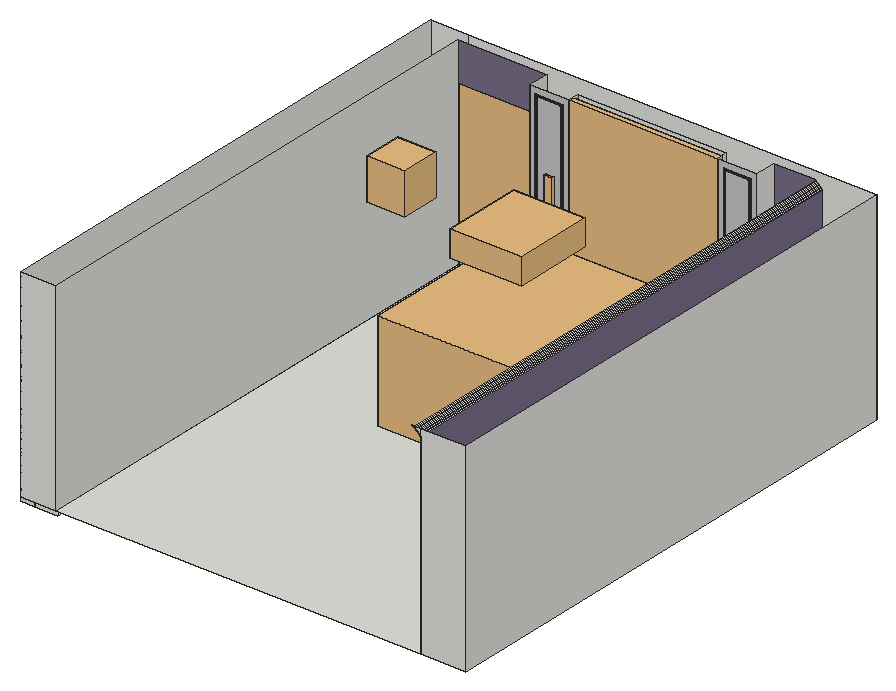
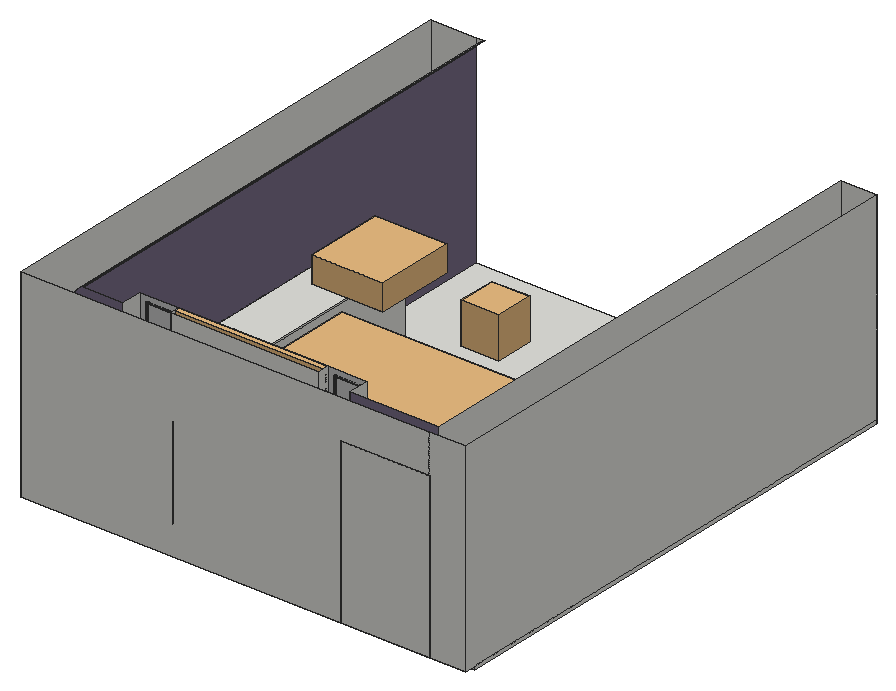
# SketchUp Ruby script. Lengths in inches.
U = 1.inch
M = Sketchup.active_model
def pt(a) = Geom::Point3d.new(a.map { |v| v * U })
def face(e, loops, mat)
  f = e.add_face(loops[0].map { |a| pt(a) })
  loops[1..].each { |l| e.add_face(l.map { |a| pt(a) }).erase! }
  f.material = f.back_material = mat if mat
  f
end
# faces: each face lists its corners as indices into pts; further lists are holes
def faces(e, pts, list, mat = nil) = list.each { |f| face(e, (f[0].is_a?(Array) ? f : [f]).map { |l| l.map { |i| pts[i] } }, mat) }
# xy, xz, yz: faces in a plane at the given z, y or x. An outline is a flat list of corners, or four numbers for a rectangle; further outlines are holes
def ring(l) = l.size == 4 ? [[l[0], l[1]], [l[2], l[1]], [l[2], l[3]], [l[0], l[3]]] : l.each_slice(2).to_a
def flat(e, list, mat, &to3) = list.each { |f| face(e, (f[0].is_a?(Array) ? f : [f]).map { |l| ring(l).map { |u, v| to3.(u, v) } }, mat) }
def xy(e, z, list, mat = nil) = flat(e, list, mat) { |x, y| [x, y, z] }
def xz(e, y, list, mat = nil) = flat(e, list, mat) { |x, z| [x, y, z] }
def yz(e, x, list, mat = nil) = flat(e, list, mat) { |y, z| [x, y, z] }
def lines(e, pts, list) = list.each { |a, b| e.add_line(pt(pts[a]), pt(pts[b])) }
# prism: a flat outline (further loops are holes) pulled along v
def prism(e, loops, v, mat = nil)
  f = face(e, loops, mat); d = Geom::Vector3d.new(v.map { |x| x * U })
  f.pushpull(f.normal.samedirection?(d) ? d.length : -d.length)
end
def box(e, o, s, mat = nil) = prism(e, [[o, [o[0] + s[0], o[1], o[2]], [o[0] + s[0], o[1] + s[1], o[2]], [o[0], o[1] + s[1], o[2]]]], [0, 0, s[2]], mat)
def at(x, y, z, deg = 0) = Geom::Transformation.translation(pt([x, y, z])) * Geom::Transformation.rotation(ORIGIN, Z_AXIS, deg.degrees)
def axes(o, x, y, z) = Geom::Transformation.new([*x, 0, *y, 0, *z, 0, *pt(o).to_a, 1])
def part(name) = M.definitions.add(name)
# library, detail: a bought-in or finely detailed component or shape, given as its bounding box
def library(name, o, s) = part(name).tap { |d| box(d.entities, o, s) }
def detail(e, o, s) = box(e.add_group.entities, o, s)
def put(e, d, t, mat = nil) = e.add_instance(d, t).tap { |i| i.material = mat if mat }
def group(e, t, mat = nil) = e.add_group.tap { |g| g.transformation = t; g.material = mat if mat }.entities
root = M.entities
M.materials.add("[0116_Lavender]").color = [230, 230, 250]
M.materials.add("[Color J01]2").color = [122, 110, 137]
M.materials.add("[Color M01]").color = [226, 226, 226]
M.materials.add("[Color M02]").color = [198, 198, 198]
M.materials.add("[Color M07]").color = [58, 58, 58]
M.materials.add("[Color M08]").color = [30, 30, 30]
c1 = library("Group\#22",[0,-0.85,0],[159.52,154.66,89.09])
c2 = library("Group\#1",[0,0,0],[152.125,5.875,206.4375])
c3 = library("Untitled (23)",[0,0,0],[36,4.39,84])
c4 = part("Group\#46")
prism(c4.entities,[[[0.55,0,1.11],[0.51,0,1.03],[0.44,0,0.97],[0.36,0,0.9375],[0.28,0,0.92],[0.19,0,0.9375],[0.11,0,0.97],[0.05,0,1.03],[0,0,1.11],[0,0,0],[0.55,0,0]]],[0,0.79,0])
c5 = part("Cabinet pull")
put(c5.entities,c4,axes([0,1.42,1.36],[0,0,-1],[1,0,0],[0,-1,0]),"[Color M08]")
g1 = group(c5.entities,at(0,1.42,1.36),"[Color M08]")
prism(g1,[[[0,-1.28,-0.57],[0,-1.32,-0.53],[0,-1.35,-0.49],[0,-1.38,-0.4375],[0,-1.4,-0.39],[0,-1.41,-0.33],[0,-1.42,-0.28],[0,-1.41,-0.22],[0,-1.4,-0.17],[0,-1.38,-0.11],[0,-1.35,-0.0625],[0,-1.32,-0.02],[0,-1.28,0.02],[0,-1.19,0.02],[0,-1.11,0],[0,-1.03,-0.05],[0,-0.97,-0.11],[0,-0.9375,-0.19],[0,-0.92,-0.28],[0,-0.9375,-0.36],[0,-0.97,-0.44],[0,-1.03,-0.51],[0,-1.11,-0.55],[0,-1.19,-0.57]]],[13.07,0,0])
put(c5.entities,c4,axes([12.28,1.42,1.36],[0,0,-1],[1,0,0],[0,-1,0]),"[Color M08]")
c6 = library("Group\#4",[0,0,0],[7.875,1.97,51.61])
c7 = library("Bathroom accessory set",[0,0,0],[18.8125,6.58,10.0625])
c8 = library("lamp",[0,0,0],[9.82,9.84,19.44])
c9 = library("Tabletop vanity mirror",[-0.04,0,0],[13.32,7.875,17.05])
c10 = library("Perfume bottle",[0,0,0],[5.52,3.68,7.92])
c11 = library("Pendant lamp Queen P0244",[-19.36,-19.5625,0],[38.72,39.125,72.84])
c12 = library("031_FANZART_Zen",[-27.59,-27.12,5.07],[46.53,51.77,17.09])
xy(root,-3.875,[[0,0,38.125,513.375]])
xy(root,0,[[0,0,14.41,513.375],[14.41,0,36.34,513.375],[36.34,0,409.59,0,409.59,513.375,359.78,513.375,359.78,491.75,319.78,491.75,319.78,502.75,167.66,502.75,167.66,491.75,127.66,491.75,127.66,524.91,36.34,524.91],[409.59,0,455.6875,0,455.6875,524.91,127.66,524.91,127.66,491.75,167.66,491.75,167.66,502.75,319.78,502.75,319.78,491.75,359.78,491.75,359.78,513.375,409.59,513.375],[0,513.375,36.34,524.91]])
xy(root,4,[[355.03,159.1875,409.59,466.85]])
xy(root,87.5625,[[355.03,159.1875,409.59,466.85]])
xy(root,89.5625,[[355.03,159.1875,409.59,466.85]])
xy(root,166.72,[[36.34,513.375,127.66,524.91]])
xy(root,200.41,[[133.68,491.52,161.63,491.52,161.625,491.75,133.6875,491.75]])
xz(root,0,[[0,-3.875,14.41,0],[14.41,-3.875,38.125,0],[0,0,36.34,206.4375],[409.59,0,455.6875,206.4375],[409.59,198.52,409.59,206.4375,400.78,206.4375,401.6875,206.01,402.57,205.53,403.43,205.01,404.25,204.4375,405.05,203.83,405.8125,203.18,406.54,202.49,407.23,201.76,407.89,201,408.5,200.2,409.07,199.38]])
xz(root,159.1875,[[355.03,4,409.59,87.5625],[355.03,87.5625,409.59,89.5625]])
xz(root,466.85,[[355.03,4,409.59,87.5625],[355.03,87.5625,409.59,89.5625]])
xz(root,491.75,[[[127.66,0,167.66,206.4375],[133.6875,6.03,161.625,200.41]],[[319.78,0,359.78,206.4375],[326.02,6.24,353.54,200.2]],[135.25,7.59,160.0625,198.84],[327.71,7.93,351.86,198.51]],"[Color M02]")
xz(root,502.75,[[167.66,0,319.78,206.4375]])
xz(root,513.375,[[0,-3.875,14.41,0]])
xz(root,513.375,[[359.78,0,409.59,0,409.59,198.52,409.07,199.38,408.5,200.2,407.89,201,407.23,201.76,406.54,202.49,405.8125,203.18,405.05,203.83,404.25,204.4375,403.43,205.01,402.57,205.53,401.6875,206.01,400.78,206.4375,359.78,206.4375],[36.34,166.72,127.66,206.4375]],"[Color J01]2")
xz(root,524.91,[[0,0,0,206.4375,38.125,206.4375,38.125,166.72,36.34,166.72,36.34,0],[36.34,0,127.66,166.72],[127.66,0,127.66,166.72,38.125,166.72,38.125,206.4375,455.6875,206.4375,455.6875,0]])
yz(root,0,[[0,-3.875,513.375,0],[0,0,524.91,206.4375]])
yz(root,14.41,[[0,-3.875,513.375,0]])
yz(root,36.34,[[0,0,524.91,0,524.91,166.72,513.375,166.72,513.375,206.4375,0,206.4375]])
yz(root,127.66,[[491.75,0,491.75,206.4375,513.375,206.4375,513.375,166.72,524.91,166.72,524.91,0]])
yz(root,167.66,[[491.75,0,502.75,206.4375]])
yz(root,319.78,[[491.75,0,502.75,206.4375]])
yz(root,355.03,[[159.1875,4,350.16,87.5625],[408.5,4,466.85,87.5625],[159.1875,87.5625,350.16,89.5625],[350.16,87.5625,408.5,89.5625],[408.5,87.5625,466.85,89.5625]])
yz(root,355.03,[[350.16,4,408.5,24.02],[350.16,24.89,408.5,44.91],[350.16,45.78,408.5,65.8],[350.16,66.67,408.5,86.39]],"[Color J01]2")
yz(root,355.03,[[350.16,24.02,408.5,24.89],[350.16,44.91,408.5,45.78],[350.16,65.8,408.5,66.67],[350.16,86.39,408.5,87.5625]],"[Color M07]")
yz(root,359.78,[[491.75,0,513.375,206.4375]])
yz(root,409.59,[[159.1875,87.5625,466.85,89.5625]])
yz(root,409.59,[[[0,0,513.375,198.52],[159.1875,4,466.85,89.5625]]],"[Color J01]2")
yz(root,455.6875,[[0,0,524.91,206.4375]])
p = [[133.68,491.52,6.02],[133.74,491.29,6.08],[133.74,491.29,200.35],[133.68,491.52,200.41],[161.63,491.52,6.02],[161.57,491.29,6.08],
  [161.63,491.52,200.41],[161.57,491.29,200.35],[133.6875,491.75,6.03],[133.6875,491.75,200.41],[161.625,491.75,6.03],[161.625,491.75,200.41],
  [133.86,491.1,6.2],[133.86,491.1,200.23],[161.45,491.1,6.2],[161.45,491.1,200.23],[134.03,490.94,6.375],[134.03,490.94,200.0625],
  [161.28,490.94,6.375],[161.28,490.94,200.0625],[326.02,491.75,6.24],[326.05,491.53,6.27],[326.05,491.53,200.17],[326.02,491.75,200.2],
  [353.54,491.75,6.24],[353.51,491.53,6.27],[327.71,491.53,6.27],[327.71,491.75,6.24],[353.54,491.75,200.2],[353.51,491.53,200.17],
  [326.13,491.33,6.35],[326.13,491.33,200.09],[327.71,491.33,6.35],[353.43,491.33,6.35],[353.43,491.33,200.09],[134.24,490.85,6.58],
  [134.24,490.85,199.85],[161.07,490.85,6.58],[161.07,490.85,199.85],[326.27,491.15,6.49],[326.27,491.15,199.95],[327.71,491.15,6.49],
  [353.3,491.15,6.49],[353.3,491.15,199.95],[326.44,491.02,6.66],[326.44,491.02,199.78],[353.12,491.02,6.66],[327.71,491.02,6.66],
  [353.12,491.02,199.78],[134.47,490.8125,6.8125],[134.47,490.8125,199.625],[160.84,490.8125,6.8125],[160.84,490.8125,199.625],[326.65,490.93,6.86],
  [326.65,490.93,199.57],[352.92,490.93,6.86],[327.71,490.93,6.86],[352.92,490.93,199.57],[134.7,490.85,7.04],[134.7,490.85,199.4],
  [160.61,490.85,7.04],[160.61,490.85,199.4],[326.86,490.91,7.08],[326.86,490.91,199.36],[352.7,490.91,7.08],[327.71,490.91,7.08],
  [352.7,490.91,199.36],[134.91,490.94,7.25],[134.91,490.94,199.1875],[160.4,490.94,7.25],[160.4,490.94,199.1875],[327.08,490.93,7.3],
  [327.08,490.93,199.14],[352.48,490.93,7.3],[327.71,490.93,7.3],[352.48,490.93,199.14],[135.08,491.1,7.42],[135.08,491.1,199.01],
  [160.23,491.1,7.42],[160.23,491.1,199.01],[327.29,491.02,7.5],[327.29,491.02,198.93],[352.28,491.02,7.5],[327.71,491.02,7.5],
  [352.28,491.02,198.93],[135.2,491.29,7.54],[135.2,491.29,198.89],[160.11,491.29,7.54],[160.11,491.29,198.89],[327.46,491.15,7.68],
  [327.46,491.15,198.76],[352.1,491.15,7.68],[327.71,491.15,7.68],[352.1,491.15,198.76],[135.26,491.52,7.6],[135.26,491.52,198.83],
  [160.05,491.52,7.6],[160.05,491.52,198.83],[135.25,491.75,7.59],[135.25,491.75,198.84],[160.0625,491.75,7.59],[160.0625,491.75,198.84],
  [327.59,491.33,7.8125],[327.59,491.33,198.625],[351.97,491.33,7.8125],[327.71,491.33,7.8125],[351.97,491.33,198.625],[327.68,491.53,7.9],
  [327.68,491.53,198.54],[327.71,491.53,7.9],[351.88,491.53,7.9],[351.88,491.53,198.54],[327.71,491.75,7.93],[327.71,491.75,198.51],
  [351.86,491.75,7.93],[351.86,491.75,198.51],[409.07,513.375,199.38],[409.59,513.375,198.52],[409.59,0,198.52],[409.07,0,199.38],
  [408.5,513.375,200.2],[408.5,0,200.2],[407.89,513.375,201],[407.89,0,201],[407.23,513.375,201.76],[407.23,0,201.76],
  [406.54,513.375,202.49],[406.54,0,202.49],[405.8125,513.375,203.18],[405.8125,0,203.18],[405.05,513.375,203.83],[405.05,0,203.83],
  [404.25,513.375,204.4375],[404.25,0,204.4375],[403.43,513.375,205.01],[403.43,0,205.01],[402.57,513.375,205.53],[402.57,0,205.53]]
faces(root,p,[[0,1,2,3],[4,5,1,0],[8,0,3,9],[10,4,0,8],[1,12,13,2],[5,14,12,1],[12,16,17,13],[14,18,16,12],
  [24,25,26,21,20,27],[32,30,21,26,25,33],[16,35,36,17],[18,37,35,16],[41,39,30,32,33,42],[42,46,47,44,39,41],[35,49,50,36],[37,51,49,35],
  [46,55,56,53,44,47],[49,58,59,50],[51,60,58,49],[55,64,65,62,53,56],[58,67,68,59],[60,69,67,58],[64,73,74,71,62,65],[67,76,77,68],
  [69,78,76,67],[73,82,83,80,71,74],[76,85,86,77],[78,87,85,76],[82,91,92,89,80,83],[85,94,95,86],[87,96,94,85],[94,98,99,95],
  [96,100,98,94],[91,104,105,102,89,92],[109,107,102,105,104,110],[112,107,109,110,114],[116,117,118,119],[103,108,111,106],[108,113,115,111],[90,103,106,93],
  [81,90,93,84],[86,95,97,88],[95,99,101,97],[72,81,84,75],[77,86,88,79],[68,77,79,70],[63,72,75,66],[59,68,70,61],
  [120,116,119,121],[50,59,61,52],[54,63,66,57],[36,50,52,38],[45,54,57,48],[40,45,48,43],[17,36,38,19],[31,40,43,34],
  [13,17,19,15],[22,31,34,29],[122,120,121,123],[2,13,15,7],[23,22,29,28],[3,2,7,6],[124,122,123,125],[126,124,125,127],
  [128,126,127,129],[130,128,129,131],[132,130,131,133],[134,132,133,135],[136,134,135,137]])
faces(root,p,[[6,7,5,4],[11,6,4,10],[7,15,14,5],[15,19,18,14],[19,38,37,18],[38,52,51,37],[52,61,60,51],[61,70,69,60],
  [70,79,78,69],[79,88,87,78],[88,97,96,87],[97,101,100,96]],"[Color M01]")
faces(root,p,[[20,21,22,23],[21,30,31,22],[30,39,40,31],[39,44,45,40],[44,53,54,45],[53,62,63,54],[62,71,72,63],[71,80,81,72],
  [80,89,90,81],[89,102,103,90],[102,107,108,103],[107,112,113,108]],"[Color M02]")
faces(root,p,[[28,29,25,24],[29,34,33,25],[34,43,42,33],[43,48,46,42],[48,57,55,46],[57,66,64,55],[66,75,73,64],[75,84,82,73],
  [84,93,91,82],[93,106,104,91],[106,111,110,104],[111,115,114,110]],"[0116_Lavender]")
put(root,c1,axes([150.38,269.97,0],[1.1342,0,0],[0,1.1342,0],[0,0,1.1342]))
put(root,c2,at(167.66,491.75,0),"[Color M02]")
put(root,c3,axes([37.06,514.75,0],[2.51667,0,0],[0,1,0],[0,0,1.9847]))
put(root,c5,at(353.61,385.24,22.65,-90))
put(root,c5,at(353.61,385.24,43.47,-90))
put(root,c5,at(353.61,385.24,64.47,-90))
put(root,c6,at(334.75,488.35,76.14))
put(root,c6,at(143.99,489.78,79.24))
put(root,c5,at(353.61,385.24,85.22,-90))
put(root,c7,axes([378.68,376.48,89.55],[0,-1.02,0],[1.02,0,0],[0,0,1.02]))
put(root,c8,axes([357.3,424.95,89.5625],[2.4674,0,0],[0,2.4674,0],[0,0,2.4674]))
put(root,c9,axes([361.2,395.92,89.5625],[0.23616,-1.33934,0],[1.33934,0.23616,0],[0,0,1.36]))
put(root,c10,axes([380.63,352.95,90.35],[0,-1.36,0],[1.36,0,0],[0,0,1.36]))
put(root,c11,axes([124.98,330.75,170.76],[1,0,0],[0,1,0],[0,0,0.58]),"[Color M01]")
put(root,c12,axes([264.65,315.21,168.89],[1.57,0,0],[0,1.57,0],[0,0,1.57]))
